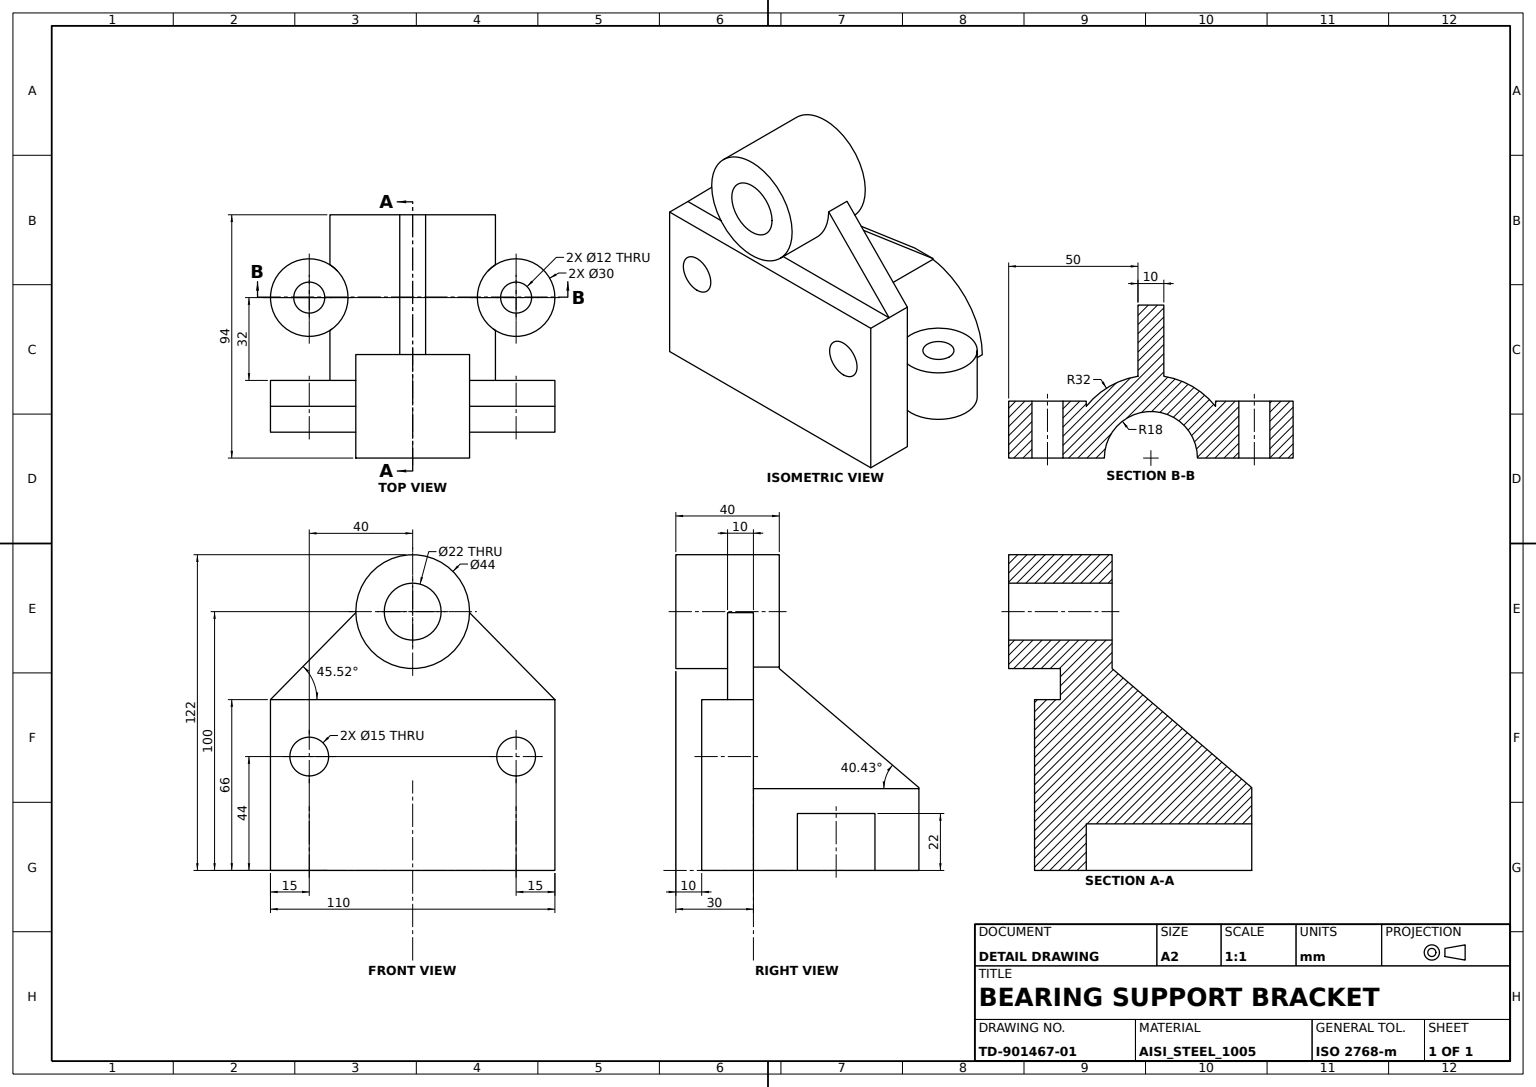
ISO-10303-21;
HEADER;
FILE_DESCRIPTION((''),'2;1');
FILE_NAME('','',(''),(''),'','','');
FILE_SCHEMA(('AUTOMOTIVE_DESIGN'));
ENDSEC;
DATA;
#1=APPLICATION_CONTEXT('');
#2=PRODUCT_CONTEXT('',#1,'mechanical');
#3=PRODUCT('','','',(#2));
#4=PRODUCT_DEFINITION_FORMATION('','',#3);
#5=PRODUCT_DEFINITION_CONTEXT('',#1,'design');
#6=PRODUCT_DEFINITION('','',#4,#5);
#7=PRODUCT_DEFINITION_SHAPE('','',#6);
#8=(LENGTH_UNIT()NAMED_UNIT(*)SI_UNIT(.MILLI.,.METRE.));
#9=(NAMED_UNIT(*)PLANE_ANGLE_UNIT()SI_UNIT($,.RADIAN.));
#10=(NAMED_UNIT(*)SI_UNIT($,.STERADIAN.)SOLID_ANGLE_UNIT());
#11=UNCERTAINTY_MEASURE_WITH_UNIT(LENGTH_MEASURE(0.005),#8,'distance_accuracy_value','');
#12=(GEOMETRIC_REPRESENTATION_CONTEXT(3)GLOBAL_UNCERTAINTY_ASSIGNED_CONTEXT((#11))GLOBAL_UNIT_ASSIGNED_CONTEXT((#8,#9,#10))REPRESENTATION_CONTEXT('',''));
#13=CARTESIAN_POINT('',(-47.5,0.,44.));
#14=VERTEX_POINT('',#13);
#15=CARTESIAN_POINT('',(-40.,0.,44.));
#16=DIRECTION('',(0.,1.,0.));
#17=DIRECTION('',(-1.,0.,0.));
#18=AXIS2_PLACEMENT_3D('',#15,#16,#17);
#19=CIRCLE('',#18,7.5);
#20=EDGE_CURVE('',#14,#14,#19,.T.);
#21=ORIENTED_EDGE('',*,*,#20,.T.);
#22=EDGE_LOOP('',(#21));
#23=FACE_BOUND('',#22,.T.);
#24=CARTESIAN_POINT('',(-40.,-20.,36.5));
#25=VERTEX_POINT('',#24);
#26=CARTESIAN_POINT('',(-40.,-20.,44.));
#27=DIRECTION('',(0.,-1.,0.));
#28=DIRECTION('',(0.,0.,-1.));
#29=AXIS2_PLACEMENT_3D('',#26,#27,#28);
#30=CIRCLE('',#29,7.5);
#31=EDGE_CURVE('',#25,#25,#30,.T.);
#32=ORIENTED_EDGE('',*,*,#31,.T.);
#33=EDGE_LOOP('',(#32));
#34=FACE_BOUND('',#33,.T.);
#35=CARTESIAN_POINT('',(-40.,-40.,44.));
#36=DIRECTION('',(0.,0.,1.));
#37=AXIS2_PLACEMENT_3D('',#35,#16,#36);
#38=CYLINDRICAL_SURFACE('',#37,7.5);
#39=ADVANCED_FACE('',(#23,#34),#38,.F.);
#40=CARTESIAN_POINT('',(32.5,0.,44.));
#41=VERTEX_POINT('',#40);
#42=CARTESIAN_POINT('',(40.,0.,44.));
#43=AXIS2_PLACEMENT_3D('',#42,#16,#17);
#44=CIRCLE('',#43,7.5);
#45=EDGE_CURVE('',#41,#41,#44,.T.);
#46=ORIENTED_EDGE('',*,*,#45,.F.);
#47=EDGE_LOOP('',(#46));
#48=FACE_BOUND('',#47,.T.);
#49=CARTESIAN_POINT('',(55.,0.,0.));
#50=VERTEX_POINT('',#49);
#51=CARTESIAN_POINT('',(55.,0.,66.));
#52=VERTEX_POINT('',#51);
#53=VECTOR('',#36,1000.);
#54=LINE('',#49,#53);
#55=EDGE_CURVE('',#50,#52,#54,.T.);
#56=ORIENTED_EDGE('',*,*,#55,.F.);
#57=CARTESIAN_POINT('',(32.,0.,0.));
#58=VERTEX_POINT('',#57);
#59=CARTESIAN_POINT('',(0.,0.,0.));
#60=DIRECTION('',(1.,0.,0.));
#61=VECTOR('',#60,1000.);
#62=LINE('',#59,#61);
#63=EDGE_CURVE('',#58,#50,#62,.T.);
#64=ORIENTED_EDGE('',*,*,#63,.F.);
#65=CARTESIAN_POINT('',(5.,0.,31.606961));
#66=VERTEX_POINT('',#65);
#67=AXIS2_PLACEMENT_3D('',#59,#27,#60);
#68=CIRCLE('',#67,32.);
#69=EDGE_CURVE('',#58,#66,#68,.T.);
#70=ORIENTED_EDGE('',*,*,#69,.T.);
#71=CARTESIAN_POINT('',(5.,0.,78.575715));
#72=VERTEX_POINT('',#71);
#73=CARTESIAN_POINT('',(5.,0.,0.));
#74=LINE('',#73,#53);
#75=EDGE_CURVE('',#66,#72,#74,.T.);
#76=ORIENTED_EDGE('',*,*,#75,.T.);
#77=CARTESIAN_POINT('',(21.996429,0.,99.603636));
#78=VERTEX_POINT('',#77);
#79=CARTESIAN_POINT('',(0.,0.,100.));
#80=AXIS2_PLACEMENT_3D('',#79,#27,#28);
#81=CIRCLE('',#80,22.);
#82=EDGE_CURVE('',#72,#78,#81,.T.);
#83=ORIENTED_EDGE('',*,*,#82,.T.);
#84=DIRECTION('',(-0.700708015,0.,0.713448161));
#85=VECTOR('',#84,1000.);
#86=LINE('',#51,#85);
#87=EDGE_CURVE('',#52,#78,#86,.T.);
#88=ORIENTED_EDGE('',*,*,#87,.F.);
#89=EDGE_LOOP('',(#56,#64,#70,#76,#83,#88));
#90=FACE_BOUND('',#89,.T.);
#91=AXIS2_PLACEMENT_3D('',#59,#27,#28);
#92=PLANE('',#91);
#93=ADVANCED_FACE('',(#48,#90),#92,.F.);
#94=CARTESIAN_POINT('',(-5.,10.,78.575715));
#95=VERTEX_POINT('',#94);
#96=CARTESIAN_POINT('',(-5.,10.,78.));
#97=VERTEX_POINT('',#96);
#98=CARTESIAN_POINT('',(-5.,10.,122.));
#99=VECTOR('',#28,1000.);
#100=LINE('',#98,#99);
#101=EDGE_CURVE('',#95,#97,#100,.T.);
#102=ORIENTED_EDGE('',*,*,#101,.T.);
#103=CARTESIAN_POINT('',(-5.,64.,32.));
#104=VERTEX_POINT('',#103);
#105=DIRECTION('',(0.,0.76124323,-0.648466456));
#106=VECTOR('',#105,1000.);
#107=LINE('',#96,#106);
#108=EDGE_CURVE('',#97,#104,#107,.T.);
#109=ORIENTED_EDGE('',*,*,#108,.T.);
#110=CARTESIAN_POINT('',(-5.,64.,31.606961));
#111=VERTEX_POINT('',#110);
#112=LINE('',#103,#99);
#113=EDGE_CURVE('',#104,#111,#112,.T.);
#114=ORIENTED_EDGE('',*,*,#113,.T.);
#115=CARTESIAN_POINT('',(-5.,0.,31.606961));
#116=VERTEX_POINT('',#115);
#117=VECTOR('',#27,1000.);
#118=LINE('',#110,#117);
#119=EDGE_CURVE('',#116,#111,#118,.F.);
#120=ORIENTED_EDGE('',*,*,#119,.F.);
#121=CARTESIAN_POINT('',(-5.,0.,78.575715));
#122=VERTEX_POINT('',#121);
#123=CARTESIAN_POINT('',(-5.,0.,0.));
#124=LINE('',#123,#53);
#125=EDGE_CURVE('',#122,#116,#124,.F.);
#126=ORIENTED_EDGE('',*,*,#125,.F.);
#127=CARTESIAN_POINT('',(-5.,-30.,78.575715));
#128=VECTOR('',#16,1000.);
#129=LINE('',#127,#128);
#130=EDGE_CURVE('',#95,#122,#129,.F.);
#131=ORIENTED_EDGE('',*,*,#130,.F.);
#132=EDGE_LOOP('',(#102,#109,#114,#120,#126,#131));
#133=FACE_BOUND('',#132,.T.);
#134=AXIS2_PLACEMENT_3D('',#123,#17,#36);
#135=PLANE('',#134);
#136=ADVANCED_FACE('',(#133),#135,.T.);
#137=CARTESIAN_POINT('',(46.,32.,22.));
#138=VERTEX_POINT('',#137);
#139=CARTESIAN_POINT('',(40.,32.,22.));
#140=AXIS2_PLACEMENT_3D('',#139,#36,#60);
#141=CIRCLE('',#140,6.);
#142=EDGE_CURVE('',#138,#138,#141,.T.);
#143=ORIENTED_EDGE('',*,*,#142,.T.);
#144=EDGE_LOOP('',(#143));
#145=FACE_BOUND('',#144,.T.);
#146=CARTESIAN_POINT('',(46.,32.,0.));
#147=VERTEX_POINT('',#146);
#148=CARTESIAN_POINT('',(40.,32.,0.));
#149=AXIS2_PLACEMENT_3D('',#148,#36,#60);
#150=CIRCLE('',#149,6.);
#151=EDGE_CURVE('',#147,#147,#150,.T.);
#152=ORIENTED_EDGE('',*,*,#151,.F.);
#153=EDGE_LOOP('',(#152));
#154=FACE_BOUND('',#153,.T.);
#155=AXIS2_PLACEMENT_3D('',#139,#28,#17);
#156=CYLINDRICAL_SURFACE('',#155,6.);
#157=ADVANCED_FACE('',(#145,#154),#156,.F.);
#158=CARTESIAN_POINT('',(-55.,-20.,66.));
#159=VERTEX_POINT('',#158);
#160=CARTESIAN_POINT('',(-55.,-20.,0.));
#161=VERTEX_POINT('',#160);
#162=LINE('',#158,#99);
#163=EDGE_CURVE('',#159,#161,#162,.T.);
#164=ORIENTED_EDGE('',*,*,#163,.F.);
#165=CARTESIAN_POINT('',(-55.,-10.,66.));
#166=VERTEX_POINT('',#165);
#167=LINE('',#158,#128);
#168=EDGE_CURVE('',#159,#166,#167,.T.);
#169=ORIENTED_EDGE('',*,*,#168,.T.);
#170=CARTESIAN_POINT('',(-55.,0.,66.));
#171=VERTEX_POINT('',#170);
#172=LINE('',#165,#128);
#173=EDGE_CURVE('',#166,#171,#172,.T.);
#174=ORIENTED_EDGE('',*,*,#173,.T.);
#175=CARTESIAN_POINT('',(-55.,0.,0.));
#176=VERTEX_POINT('',#175);
#177=LINE('',#170,#99);
#178=EDGE_CURVE('',#171,#176,#177,.T.);
#179=ORIENTED_EDGE('',*,*,#178,.T.);
#180=LINE('',#160,#128);
#181=EDGE_CURVE('',#161,#176,#180,.T.);
#182=ORIENTED_EDGE('',*,*,#181,.F.);
#183=EDGE_LOOP('',(#164,#169,#174,#179,#182));
#184=FACE_BOUND('',#183,.T.);
#185=AXIS2_PLACEMENT_3D('',#158,#60,#28);
#186=PLANE('',#185);
#187=ADVANCED_FACE('',(#184),#186,.F.);
#188=CARTESIAN_POINT('',(55.,32.,22.));
#189=VERTEX_POINT('',#188);
#190=CIRCLE('',#140,15.);
#191=EDGE_CURVE('',#189,#189,#190,.T.);
#192=ORIENTED_EDGE('',*,*,#191,.F.);
#193=EDGE_LOOP('',(#192));
#194=FACE_BOUND('',#193,.T.);
#195=CARTESIAN_POINT('',(32.,19.311422,0.));
#196=VERTEX_POINT('',#195);
#197=CARTESIAN_POINT('',(32.,44.688578,0.));
#198=VERTEX_POINT('',#197);
#199=CARTESIAN_POINT('',(32.,19.311422,2.323278));
#200=CARTESIAN_POINT('',(31.622894,19.530388,5.758145));
#201=CARTESIAN_POINT('',(30.408776,20.440017,10.153327));
#202=CARTESIAN_POINT('',(29.203867,21.530402,13.212042));
#203=CARTESIAN_POINT('',(27.790535,23.173449,15.953094));
#204=CARTESIAN_POINT('',(26.3726,25.499915,18.171363));
#205=CARTESIAN_POINT('',(25.27973,28.517172,19.632022));
#206=CARTESIAN_POINT('',(24.861218,31.987396,20.145077));
#207=CARTESIAN_POINT('',(25.275422,35.469381,19.637547));
#208=CARTESIAN_POINT('',(26.370681,38.496812,18.174227));
#209=CARTESIAN_POINT('',(27.789355,40.825096,15.955387));
#210=CARTESIAN_POINT('',(29.204485,42.470253,13.210549));
#211=CARTESIAN_POINT('',(30.407716,43.559061,10.156487));
#212=CARTESIAN_POINT('',(31.623653,44.470254,5.755501));
#213=CARTESIAN_POINT('',(32.,44.688578,2.324193));
#214=B_SPLINE_CURVE_WITH_KNOTS('',3,(#195,#199,#200,#201,#202,#203,#204,#205,#206,#207,#208,#209,#210,#211,#212,#213,#197),.UNSPECIFIED.,.F.,.F.,(4,1,1,1,1,1,1,1,1,1,1,1,1,1,4),(0.,0.006898826,0.010348238,0.013797651,0.017247064,0.020696477,0.024145889,0.027595302,0.031044715,0.034494128,0.03794354,0.041392953,0.044842366,0.048291779,0.055190604),.UNSPECIFIED.);
#215=EDGE_CURVE('',#196,#198,#214,.T.);
#216=ORIENTED_EDGE('',*,*,#215,.F.);
#217=CIRCLE('',#149,15.);
#218=EDGE_CURVE('',#196,#198,#217,.T.);
#219=ORIENTED_EDGE('',*,*,#218,.T.);
#220=EDGE_LOOP('',(#216,#219));
#221=FACE_BOUND('',#220,.T.);
#222=CYLINDRICAL_SURFACE('',#155,15.);
#223=ADVANCED_FACE('',(#194,#221),#222,.T.);
#224=CARTESIAN_POINT('',(5.,10.,78.));
#225=VERTEX_POINT('',#224);
#226=CARTESIAN_POINT('',(5.,64.,32.));
#227=VERTEX_POINT('',#226);
#228=LINE('',#224,#106);
#229=EDGE_CURVE('',#225,#227,#228,.T.);
#230=ORIENTED_EDGE('',*,*,#229,.T.);
#231=VECTOR('',#17,1000.);
#232=LINE('',#226,#231);
#233=EDGE_CURVE('',#227,#104,#232,.T.);
#234=ORIENTED_EDGE('',*,*,#233,.T.);
#235=ORIENTED_EDGE('',*,*,#108,.F.);
#236=LINE('',#224,#231);
#237=EDGE_CURVE('',#225,#97,#236,.T.);
#238=ORIENTED_EDGE('',*,*,#237,.F.);
#239=EDGE_LOOP('',(#230,#234,#235,#238));
#240=FACE_BOUND('',#239,.T.);
#241=DIRECTION('',(0.,0.648466456,0.76124323));
#242=DIRECTION('',(0.,-0.76124323,0.648466456));
#243=AXIS2_PLACEMENT_3D('',#224,#241,#242);
#244=PLANE('',#243);
#245=ADVANCED_FACE('',(#240),#244,.T.);
#246=CARTESIAN_POINT('',(-34.,32.,0.));
#247=VERTEX_POINT('',#246);
#248=CARTESIAN_POINT('',(-40.,32.,0.));
#249=AXIS2_PLACEMENT_3D('',#248,#36,#60);
#250=CIRCLE('',#249,6.);
#251=EDGE_CURVE('',#247,#247,#250,.T.);
#252=ORIENTED_EDGE('',*,*,#251,.T.);
#253=EDGE_LOOP('',(#252));
#254=FACE_BOUND('',#253,.T.);
#255=CARTESIAN_POINT('',(18.,64.,0.));
#256=VERTEX_POINT('',#255);
#257=CARTESIAN_POINT('',(32.,64.,0.));
#258=VERTEX_POINT('',#257);
#259=LINE('',#255,#61);
#260=EDGE_CURVE('',#256,#258,#259,.T.);
#261=ORIENTED_EDGE('',*,*,#260,.T.);
#262=LINE('',#257,#117);
#263=EDGE_CURVE('',#258,#198,#262,.T.);
#264=ORIENTED_EDGE('',*,*,#263,.T.);
#265=ORIENTED_EDGE('',*,*,#218,.F.);
#266=EDGE_CURVE('',#196,#58,#262,.T.);
#267=ORIENTED_EDGE('',*,*,#266,.T.);
#268=ORIENTED_EDGE('',*,*,#63,.T.);
#269=CARTESIAN_POINT('',(55.,-20.,0.));
#270=VERTEX_POINT('',#269);
#271=LINE('',#269,#128);
#272=EDGE_CURVE('',#270,#50,#271,.T.);
#273=ORIENTED_EDGE('',*,*,#272,.F.);
#274=LINE('',#160,#61);
#275=EDGE_CURVE('',#161,#270,#274,.T.);
#276=ORIENTED_EDGE('',*,*,#275,.F.);
#277=ORIENTED_EDGE('',*,*,#181,.T.);
#278=CARTESIAN_POINT('',(-32.,0.,0.));
#279=VERTEX_POINT('',#278);
#280=EDGE_CURVE('',#176,#279,#62,.T.);
#281=ORIENTED_EDGE('',*,*,#280,.T.);
#282=CARTESIAN_POINT('',(-32.,19.311422,0.));
#283=VERTEX_POINT('',#282);
#284=CARTESIAN_POINT('',(-32.,64.,0.));
#285=LINE('',#284,#117);
#286=EDGE_CURVE('',#279,#283,#285,.F.);
#287=ORIENTED_EDGE('',*,*,#286,.T.);
#288=CARTESIAN_POINT('',(-32.,44.688578,0.));
#289=VERTEX_POINT('',#288);
#290=CIRCLE('',#249,15.);
#291=EDGE_CURVE('',#289,#283,#290,.T.);
#292=ORIENTED_EDGE('',*,*,#291,.F.);
#293=VERTEX_POINT('',#284);
#294=EDGE_CURVE('',#289,#293,#285,.F.);
#295=ORIENTED_EDGE('',*,*,#294,.T.);
#296=CARTESIAN_POINT('',(-18.,64.,0.));
#297=VERTEX_POINT('',#296);
#298=LINE('',#284,#61);
#299=EDGE_CURVE('',#293,#297,#298,.T.);
#300=ORIENTED_EDGE('',*,*,#299,.T.);
#301=CARTESIAN_POINT('',(-18.,0.,0.));
#302=VERTEX_POINT('',#301);
#303=LINE('',#296,#117);
#304=EDGE_CURVE('',#297,#302,#303,.T.);
#305=ORIENTED_EDGE('',*,*,#304,.T.);
#306=CARTESIAN_POINT('',(18.,0.,0.));
#307=VERTEX_POINT('',#306);
#308=EDGE_CURVE('',#302,#307,#62,.T.);
#309=ORIENTED_EDGE('',*,*,#308,.T.);
#310=LINE('',#255,#117);
#311=EDGE_CURVE('',#307,#256,#310,.F.);
#312=ORIENTED_EDGE('',*,*,#311,.T.);
#313=EDGE_LOOP('',(#261,#264,#265,#267,#268,#273,#276,#277,#281,#287,#292,#295,#300,#305,#309,#312));
#314=FACE_BOUND('',#313,.T.);
#315=ORIENTED_EDGE('',*,*,#151,.T.);
#316=EDGE_LOOP('',(#315));
#317=FACE_BOUND('',#316,.T.);
#318=CARTESIAN_POINT('',(0.,-20.,0.));
#319=AXIS2_PLACEMENT_3D('',#318,#36,#60);
#320=PLANE('',#319);
#321=ADVANCED_FACE('',(#254,#314,#317),#320,.F.);
#322=CARTESIAN_POINT('',(5.,64.,31.606961));
#323=VERTEX_POINT('',#322);
#324=LINE('',#322,#117);
#325=EDGE_CURVE('',#323,#66,#324,.T.);
#326=ORIENTED_EDGE('',*,*,#325,.T.);
#327=ORIENTED_EDGE('',*,*,#69,.F.);
#328=ORIENTED_EDGE('',*,*,#266,.F.);
#329=ORIENTED_EDGE('',*,*,#215,.T.);
#330=ORIENTED_EDGE('',*,*,#263,.F.);
#331=CARTESIAN_POINT('',(0.,64.,0.));
#332=AXIS2_PLACEMENT_3D('',#331,#27,#60);
#333=CIRCLE('',#332,32.);
#334=EDGE_CURVE('',#258,#323,#333,.T.);
#335=ORIENTED_EDGE('',*,*,#334,.T.);
#336=EDGE_LOOP('',(#326,#327,#328,#329,#330,#335));
#337=FACE_BOUND('',#336,.T.);
#338=AXIS2_PLACEMENT_3D('',#331,#27,#28);
#339=CYLINDRICAL_SURFACE('',#338,32.);
#340=ADVANCED_FACE('',(#337),#339,.T.);
#341=AXIS2_PLACEMENT_3D('',#59,#16,#60);
#342=CIRCLE('',#341,18.);
#343=EDGE_CURVE('',#302,#307,#342,.T.);
#344=ORIENTED_EDGE('',*,*,#343,.T.);
#345=ORIENTED_EDGE('',*,*,#308,.F.);
#346=EDGE_LOOP('',(#344,#345));
#347=FACE_BOUND('',#346,.T.);
#348=ADVANCED_FACE('',(#347),#92,.F.);
#349=ORIENTED_EDGE('',*,*,#191,.T.);
#350=EDGE_LOOP('',(#349));
#351=FACE_BOUND('',#350,.T.);
#352=ORIENTED_EDGE('',*,*,#142,.F.);
#353=EDGE_LOOP('',(#352));
#354=FACE_BOUND('',#353,.T.);
#355=PLANE('',#140);
#356=ADVANCED_FACE('',(#351,#354),#355,.T.);
#357=ORIENTED_EDGE('',*,*,#251,.F.);
#358=EDGE_LOOP('',(#357));
#359=FACE_BOUND('',#358,.T.);
#360=CARTESIAN_POINT('',(-34.,32.,22.));
#361=VERTEX_POINT('',#360);
#362=CARTESIAN_POINT('',(-40.,32.,22.));
#363=AXIS2_PLACEMENT_3D('',#362,#36,#60);
#364=CIRCLE('',#363,6.);
#365=EDGE_CURVE('',#361,#361,#364,.T.);
#366=ORIENTED_EDGE('',*,*,#365,.T.);
#367=EDGE_LOOP('',(#366));
#368=FACE_BOUND('',#367,.T.);
#369=AXIS2_PLACEMENT_3D('',#362,#28,#17);
#370=CYLINDRICAL_SURFACE('',#369,6.);
#371=ADVANCED_FACE('',(#359,#368),#370,.F.);
#372=ORIENTED_EDGE('',*,*,#343,.F.);
#373=ORIENTED_EDGE('',*,*,#304,.F.);
#374=AXIS2_PLACEMENT_3D('',#331,#16,#60);
#375=CIRCLE('',#374,18.);
#376=EDGE_CURVE('',#297,#256,#375,.T.);
#377=ORIENTED_EDGE('',*,*,#376,.T.);
#378=ORIENTED_EDGE('',*,*,#311,.F.);
#379=EDGE_LOOP('',(#372,#373,#377,#378));
#380=FACE_BOUND('',#379,.T.);
#381=CYLINDRICAL_SURFACE('',#338,18.);
#382=ADVANCED_FACE('',(#380),#381,.F.);
#383=CARTESIAN_POINT('',(40.,-20.,36.5));
#384=VERTEX_POINT('',#383);
#385=CARTESIAN_POINT('',(40.,-20.,44.));
#386=AXIS2_PLACEMENT_3D('',#385,#27,#28);
#387=CIRCLE('',#386,7.5);
#388=EDGE_CURVE('',#384,#384,#387,.T.);
#389=ORIENTED_EDGE('',*,*,#388,.T.);
#390=EDGE_LOOP('',(#389));
#391=FACE_BOUND('',#390,.T.);
#392=ORIENTED_EDGE('',*,*,#45,.T.);
#393=EDGE_LOOP('',(#392));
#394=FACE_BOUND('',#393,.T.);
#395=CARTESIAN_POINT('',(40.,-40.,44.));
#396=AXIS2_PLACEMENT_3D('',#395,#16,#36);
#397=CYLINDRICAL_SURFACE('',#396,7.5);
#398=ADVANCED_FACE('',(#391,#394),#397,.F.);
#399=ORIENTED_EDGE('',*,*,#31,.F.);
#400=EDGE_LOOP('',(#399));
#401=FACE_BOUND('',#400,.T.);
#402=CARTESIAN_POINT('',(55.,-20.,66.));
#403=VERTEX_POINT('',#402);
#404=LINE('',#269,#53);
#405=EDGE_CURVE('',#270,#403,#404,.T.);
#406=ORIENTED_EDGE('',*,*,#405,.T.);
#407=LINE('',#402,#231);
#408=EDGE_CURVE('',#403,#159,#407,.T.);
#409=ORIENTED_EDGE('',*,*,#408,.T.);
#410=ORIENTED_EDGE('',*,*,#163,.T.);
#411=ORIENTED_EDGE('',*,*,#275,.T.);
#412=EDGE_LOOP('',(#406,#409,#410,#411));
#413=FACE_BOUND('',#412,.T.);
#414=ORIENTED_EDGE('',*,*,#388,.F.);
#415=EDGE_LOOP('',(#414));
#416=FACE_BOUND('',#415,.T.);
#417=AXIS2_PLACEMENT_3D('',#318,#27,#28);
#418=PLANE('',#417);
#419=ADVANCED_FACE('',(#401,#413,#416),#418,.T.);
#420=CARTESIAN_POINT('',(-21.996429,-10.,99.603636));
#421=VERTEX_POINT('',#420);
#422=CARTESIAN_POINT('',(-21.996429,0.,99.603636));
#423=VERTEX_POINT('',#422);
#424=CARTESIAN_POINT('',(-21.996429,-30.,99.603636));
#425=LINE('',#424,#128);
#426=EDGE_CURVE('',#421,#423,#425,.T.);
#427=ORIENTED_EDGE('',*,*,#426,.T.);
#428=CARTESIAN_POINT('',(0.,0.,122.));
#429=DIRECTION('',(-0.700708015,0.,-0.713448161));
#430=VECTOR('',#429,1000.);
#431=LINE('',#428,#430);
#432=EDGE_CURVE('',#423,#171,#431,.T.);
#433=ORIENTED_EDGE('',*,*,#432,.T.);
#434=ORIENTED_EDGE('',*,*,#173,.F.);
#435=CARTESIAN_POINT('',(0.,-10.,122.));
#436=LINE('',#435,#430);
#437=EDGE_CURVE('',#421,#166,#436,.T.);
#438=ORIENTED_EDGE('',*,*,#437,.F.);
#439=EDGE_LOOP('',(#427,#433,#434,#438));
#440=FACE_BOUND('',#439,.T.);
#441=DIRECTION('',(0.713448161,0.,-0.700708015));
#442=AXIS2_PLACEMENT_3D('',#435,#441,#429);
#443=PLANE('',#442);
#444=ADVANCED_FACE('',(#440),#443,.F.);
#445=CARTESIAN_POINT('',(5.,10.,78.575715));
#446=VERTEX_POINT('',#445);
#447=CARTESIAN_POINT('',(5.,10.,122.));
#448=LINE('',#447,#99);
#449=EDGE_CURVE('',#446,#225,#448,.T.);
#450=ORIENTED_EDGE('',*,*,#449,.T.);
#451=ORIENTED_EDGE('',*,*,#237,.T.);
#452=ORIENTED_EDGE('',*,*,#101,.F.);
#453=CARTESIAN_POINT('',(0.,10.,100.));
#454=AXIS2_PLACEMENT_3D('',#453,#16,#17);
#455=CIRCLE('',#454,22.);
#456=EDGE_CURVE('',#95,#446,#455,.T.);
#457=ORIENTED_EDGE('',*,*,#456,.T.);
#458=EDGE_LOOP('',(#450,#451,#452,#457));
#459=FACE_BOUND('',#458,.T.);
#460=CARTESIAN_POINT('',(11.,10.,100.));
#461=VERTEX_POINT('',#460);
#462=AXIS2_PLACEMENT_3D('',#453,#16,#60);
#463=CIRCLE('',#462,11.);
#464=EDGE_CURVE('',#461,#461,#463,.T.);
#465=ORIENTED_EDGE('',*,*,#464,.F.);
#466=EDGE_LOOP('',(#465));
#467=FACE_BOUND('',#466,.T.);
#468=AXIS2_PLACEMENT_3D('',#453,#16,#36);
#469=PLANE('',#468);
#470=ADVANCED_FACE('',(#459,#467),#469,.T.);
#471=ORIENTED_EDGE('',*,*,#449,.F.);
#472=CARTESIAN_POINT('',(5.,-30.,78.575715));
#473=LINE('',#472,#128);
#474=EDGE_CURVE('',#72,#446,#473,.T.);
#475=ORIENTED_EDGE('',*,*,#474,.F.);
#476=ORIENTED_EDGE('',*,*,#75,.F.);
#477=ORIENTED_EDGE('',*,*,#325,.F.);
#478=LINE('',#226,#99);
#479=EDGE_CURVE('',#227,#323,#478,.T.);
#480=ORIENTED_EDGE('',*,*,#479,.F.);
#481=ORIENTED_EDGE('',*,*,#229,.F.);
#482=EDGE_LOOP('',(#471,#475,#476,#477,#480,#481));
#483=FACE_BOUND('',#482,.T.);
#484=AXIS2_PLACEMENT_3D('',#73,#17,#36);
#485=PLANE('',#484);
#486=ADVANCED_FACE('',(#483),#485,.F.);
#487=CARTESIAN_POINT('',(-25.,32.,22.));
#488=VERTEX_POINT('',#487);
#489=CIRCLE('',#363,15.);
#490=EDGE_CURVE('',#488,#488,#489,.T.);
#491=ORIENTED_EDGE('',*,*,#490,.T.);
#492=EDGE_LOOP('',(#491));
#493=FACE_BOUND('',#492,.T.);
#494=ORIENTED_EDGE('',*,*,#365,.F.);
#495=EDGE_LOOP('',(#494));
#496=FACE_BOUND('',#495,.T.);
#497=PLANE('',#363);
#498=ADVANCED_FACE('',(#493,#496),#497,.T.);
#499=CARTESIAN_POINT('',(55.,-10.,66.));
#500=VERTEX_POINT('',#499);
#501=LINE('',#165,#61);
#502=EDGE_CURVE('',#166,#500,#501,.T.);
#503=ORIENTED_EDGE('',*,*,#502,.F.);
#504=ORIENTED_EDGE('',*,*,#168,.F.);
#505=ORIENTED_EDGE('',*,*,#408,.F.);
#506=LINE('',#402,#128);
#507=EDGE_CURVE('',#403,#500,#506,.T.);
#508=ORIENTED_EDGE('',*,*,#507,.T.);
#509=EDGE_LOOP('',(#503,#504,#505,#508));
#510=FACE_BOUND('',#509,.T.);
#511=AXIS2_PLACEMENT_3D('',#402,#28,#17);
#512=PLANE('',#511);
#513=ADVANCED_FACE('',(#510),#512,.F.);
#514=ORIENTED_EDGE('',*,*,#464,.T.);
#515=EDGE_LOOP('',(#514));
#516=FACE_BOUND('',#515,.T.);
#517=CARTESIAN_POINT('',(11.,-30.,100.));
#518=VERTEX_POINT('',#517);
#519=CARTESIAN_POINT('',(0.,-30.,100.));
#520=AXIS2_PLACEMENT_3D('',#519,#16,#60);
#521=CIRCLE('',#520,11.);
#522=EDGE_CURVE('',#518,#518,#521,.T.);
#523=ORIENTED_EDGE('',*,*,#522,.F.);
#524=EDGE_LOOP('',(#523));
#525=FACE_BOUND('',#524,.T.);
#526=AXIS2_PLACEMENT_3D('',#519,#16,#36);
#527=CYLINDRICAL_SURFACE('',#526,11.);
#528=ADVANCED_FACE('',(#516,#525),#527,.F.);
#529=LINE('',#499,#128);
#530=EDGE_CURVE('',#500,#52,#529,.T.);
#531=ORIENTED_EDGE('',*,*,#530,.F.);
#532=ORIENTED_EDGE('',*,*,#507,.F.);
#533=ORIENTED_EDGE('',*,*,#405,.F.);
#534=ORIENTED_EDGE('',*,*,#272,.T.);
#535=ORIENTED_EDGE('',*,*,#55,.T.);
#536=EDGE_LOOP('',(#531,#532,#533,#534,#535));
#537=FACE_BOUND('',#536,.T.);
#538=AXIS2_PLACEMENT_3D('',#269,#17,#36);
#539=PLANE('',#538);
#540=ADVANCED_FACE('',(#537),#539,.F.);
#541=CARTESIAN_POINT('',(-22.,-30.,100.));
#542=VERTEX_POINT('',#541);
#543=AXIS2_PLACEMENT_3D('',#519,#16,#17);
#544=CIRCLE('',#543,22.);
#545=EDGE_CURVE('',#542,#542,#544,.T.);
#546=ORIENTED_EDGE('',*,*,#545,.F.);
#547=EDGE_LOOP('',(#546));
#548=FACE_BOUND('',#547,.T.);
#549=ORIENTED_EDGE('',*,*,#522,.T.);
#550=EDGE_LOOP('',(#549));
#551=FACE_BOUND('',#550,.T.);
#552=PLANE('',#526);
#553=ADVANCED_FACE('',(#548,#551),#552,.F.);
#554=ORIENTED_EDGE('',*,*,#334,.F.);
#555=ORIENTED_EDGE('',*,*,#260,.F.);
#556=ORIENTED_EDGE('',*,*,#376,.F.);
#557=ORIENTED_EDGE('',*,*,#299,.F.);
#558=EDGE_CURVE('',#111,#293,#333,.T.);
#559=ORIENTED_EDGE('',*,*,#558,.F.);
#560=ORIENTED_EDGE('',*,*,#113,.F.);
#561=ORIENTED_EDGE('',*,*,#233,.F.);
#562=ORIENTED_EDGE('',*,*,#479,.T.);
#563=EDGE_LOOP('',(#554,#555,#556,#557,#559,#560,#561,#562));
#564=FACE_BOUND('',#563,.T.);
#565=AXIS2_PLACEMENT_3D('',#331,#16,#36);
#566=PLANE('',#565);
#567=ADVANCED_FACE('',(#564),#566,.T.);
#568=ORIENTED_EDGE('',*,*,#119,.T.);
#569=ORIENTED_EDGE('',*,*,#558,.T.);
#570=ORIENTED_EDGE('',*,*,#294,.F.);
#571=CARTESIAN_POINT('',(-32.,44.688578,2.323278));
#572=CARTESIAN_POINT('',(-31.622894,44.469612,5.758145));
#573=CARTESIAN_POINT('',(-30.408776,43.559983,10.153327));
#574=CARTESIAN_POINT('',(-29.203867,42.469598,13.212042));
#575=CARTESIAN_POINT('',(-27.790535,40.826551,15.953094));
#576=CARTESIAN_POINT('',(-26.3726,38.500085,18.171363));
#577=CARTESIAN_POINT('',(-25.27973,35.482828,19.632022));
#578=CARTESIAN_POINT('',(-24.861218,32.012604,20.145077));
#579=CARTESIAN_POINT('',(-25.275422,28.530619,19.637547));
#580=CARTESIAN_POINT('',(-26.370681,25.503188,18.174227));
#581=CARTESIAN_POINT('',(-27.789355,23.174904,15.955387));
#582=CARTESIAN_POINT('',(-29.204485,21.529747,13.210549));
#583=CARTESIAN_POINT('',(-30.407716,20.440939,10.156487));
#584=CARTESIAN_POINT('',(-31.623653,19.529746,5.755501));
#585=CARTESIAN_POINT('',(-32.,19.311422,2.324193));
#586=B_SPLINE_CURVE_WITH_KNOTS('',3,(#288,#571,#572,#573,#574,#575,#576,#577,#578,#579,#580,#581,#582,#583,#584,#585,#282),.UNSPECIFIED.,.F.,.F.,(4,1,1,1,1,1,1,1,1,1,1,1,1,1,4),(0.,0.006898826,0.010348238,0.013797651,0.017247064,0.020696477,0.024145889,0.027595302,0.031044715,0.034494128,0.03794354,0.041392953,0.044842366,0.048291779,0.055190604),.UNSPECIFIED.);
#587=EDGE_CURVE('',#289,#283,#586,.T.);
#588=ORIENTED_EDGE('',*,*,#587,.T.);
#589=ORIENTED_EDGE('',*,*,#286,.F.);
#590=EDGE_CURVE('',#116,#279,#68,.T.);
#591=ORIENTED_EDGE('',*,*,#590,.F.);
#592=EDGE_LOOP('',(#568,#569,#570,#588,#589,#591));
#593=FACE_BOUND('',#592,.T.);
#594=ADVANCED_FACE('',(#593),#339,.T.);
#595=ORIENTED_EDGE('',*,*,#82,.F.);
#596=ORIENTED_EDGE('',*,*,#474,.T.);
#597=ORIENTED_EDGE('',*,*,#456,.F.);
#598=ORIENTED_EDGE('',*,*,#130,.T.);
#599=EDGE_CURVE('',#423,#122,#81,.T.);
#600=ORIENTED_EDGE('',*,*,#599,.F.);
#601=ORIENTED_EDGE('',*,*,#426,.F.);
#602=CARTESIAN_POINT('',(21.996429,-10.,99.603636));
#603=VERTEX_POINT('',#602);
#604=CARTESIAN_POINT('',(0.,-10.,100.));
#605=AXIS2_PLACEMENT_3D('',#604,#16,#36);
#606=CIRCLE('',#605,22.);
#607=EDGE_CURVE('',#603,#421,#606,.T.);
#608=ORIENTED_EDGE('',*,*,#607,.F.);
#609=CARTESIAN_POINT('',(21.996429,-30.,99.603636));
#610=LINE('',#609,#128);
#611=EDGE_CURVE('',#78,#603,#610,.F.);
#612=ORIENTED_EDGE('',*,*,#611,.F.);
#613=EDGE_LOOP('',(#595,#596,#597,#598,#600,#601,#608,#612));
#614=FACE_BOUND('',#613,.T.);
#615=ORIENTED_EDGE('',*,*,#545,.T.);
#616=EDGE_LOOP('',(#615));
#617=FACE_BOUND('',#616,.T.);
#618=CYLINDRICAL_SURFACE('',#526,22.);
#619=ADVANCED_FACE('',(#614,#617),#618,.T.);
#620=LINE('',#499,#85);
#621=EDGE_CURVE('',#500,#603,#620,.T.);
#622=ORIENTED_EDGE('',*,*,#621,.F.);
#623=ORIENTED_EDGE('',*,*,#530,.T.);
#624=ORIENTED_EDGE('',*,*,#87,.T.);
#625=ORIENTED_EDGE('',*,*,#611,.T.);
#626=EDGE_LOOP('',(#622,#623,#624,#625));
#627=FACE_BOUND('',#626,.T.);
#628=DIRECTION('',(-0.713448161,0.,-0.700708015));
#629=AXIS2_PLACEMENT_3D('',#499,#628,#84);
#630=PLANE('',#629);
#631=ADVANCED_FACE('',(#627),#630,.F.);
#632=ORIENTED_EDGE('',*,*,#291,.T.);
#633=ORIENTED_EDGE('',*,*,#587,.F.);
#634=EDGE_LOOP('',(#632,#633));
#635=FACE_BOUND('',#634,.T.);
#636=ORIENTED_EDGE('',*,*,#490,.F.);
#637=EDGE_LOOP('',(#636));
#638=FACE_BOUND('',#637,.T.);
#639=CYLINDRICAL_SURFACE('',#369,15.);
#640=ADVANCED_FACE('',(#635,#638),#639,.T.);
#641=ORIENTED_EDGE('',*,*,#280,.F.);
#642=ORIENTED_EDGE('',*,*,#178,.F.);
#643=ORIENTED_EDGE('',*,*,#432,.F.);
#644=ORIENTED_EDGE('',*,*,#599,.T.);
#645=ORIENTED_EDGE('',*,*,#125,.T.);
#646=ORIENTED_EDGE('',*,*,#590,.T.);
#647=EDGE_LOOP('',(#641,#642,#643,#644,#645,#646));
#648=FACE_BOUND('',#647,.T.);
#649=ORIENTED_EDGE('',*,*,#20,.F.);
#650=EDGE_LOOP('',(#649));
#651=FACE_BOUND('',#650,.T.);
#652=ADVANCED_FACE('',(#648,#651),#92,.F.);
#653=ORIENTED_EDGE('',*,*,#607,.T.);
#654=ORIENTED_EDGE('',*,*,#437,.T.);
#655=ORIENTED_EDGE('',*,*,#502,.T.);
#656=ORIENTED_EDGE('',*,*,#621,.T.);
#657=EDGE_LOOP('',(#653,#654,#655,#656));
#658=FACE_BOUND('',#657,.T.);
#659=CARTESIAN_POINT('',(0.,-10.,0.));
#660=AXIS2_PLACEMENT_3D('',#659,#16,#36);
#661=PLANE('',#660);
#662=ADVANCED_FACE('',(#658),#661,.F.);
#663=CLOSED_SHELL('',(#39,#93,#136,#157,#187,#223,#245,#321,#340,#348,#356,#371,#382,#398,#419,#444,#470,#486,#498,#513,#528,#540,#553,#567,#594,#619,#631,#640,#652,#662));
#664=MANIFOLD_SOLID_BREP('',#663);
#665=ADVANCED_BREP_SHAPE_REPRESENTATION('',(#664),#12);
#666=SHAPE_DEFINITION_REPRESENTATION(#7,#665);
ENDSEC;
END-ISO-10303-21;
